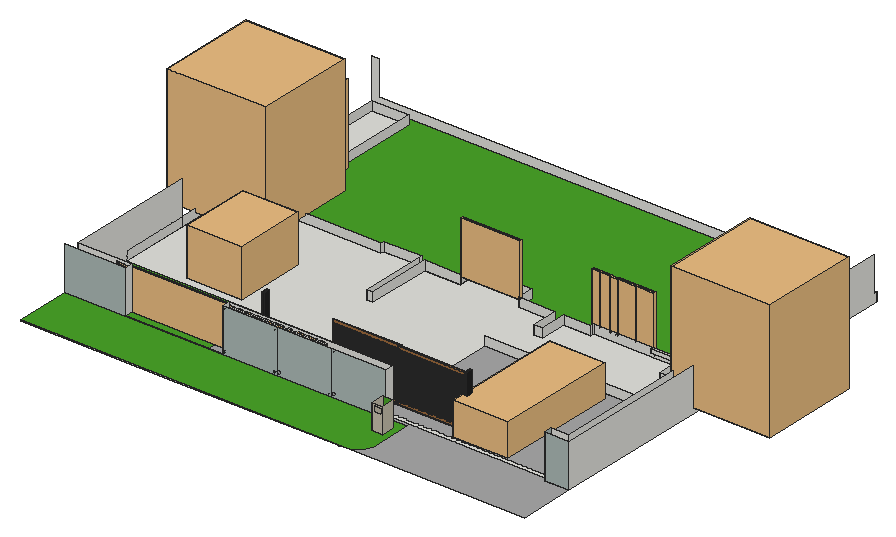
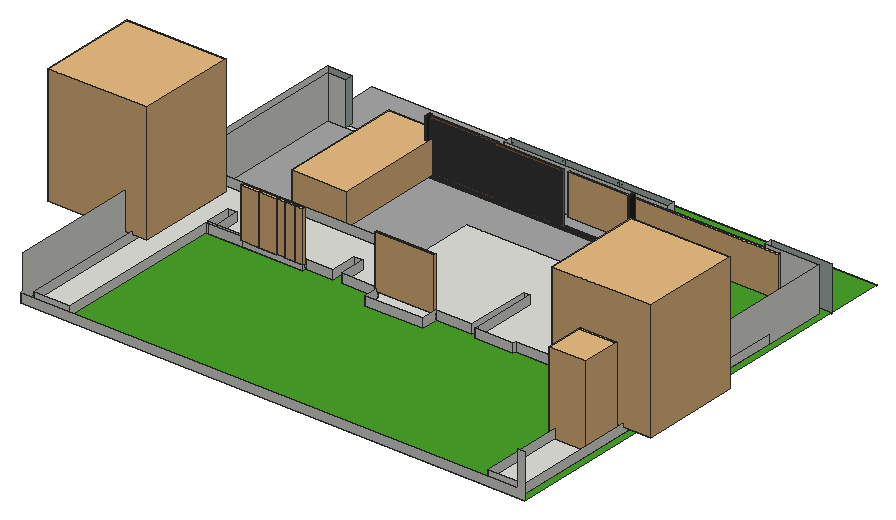
# SketchUp Ruby script. Lengths in inches.
U = 1.inch
M = Sketchup.active_model
def pt(a) = Geom::Point3d.new(a.map { |v| v * U })
def face(e, loops, mat)
  f = e.add_face(loops[0].map { |a| pt(a) })
  loops[1..].each { |l| e.add_face(l.map { |a| pt(a) }).erase! }
  f.material = f.back_material = mat if mat
  f
end
# faces: each face lists its corners as indices into pts; further lists are holes
def faces(e, pts, list, mat = nil) = list.each { |f| face(e, (f[0].is_a?(Array) ? f : [f]).map { |l| l.map { |i| pts[i] } }, mat) }
# xy, xz, yz: faces in a plane at the given z, y or x. An outline is a flat list of corners, or four numbers for a rectangle; further outlines are holes
def ring(l) = l.size == 4 ? [[l[0], l[1]], [l[2], l[1]], [l[2], l[3]], [l[0], l[3]]] : l.each_slice(2).to_a
def flat(e, list, mat, &to3) = list.each { |f| face(e, (f[0].is_a?(Array) ? f : [f]).map { |l| ring(l).map { |u, v| to3.(u, v) } }, mat) }
def xy(e, z, list, mat = nil) = flat(e, list, mat) { |x, y| [x, y, z] }
def xz(e, y, list, mat = nil) = flat(e, list, mat) { |x, z| [x, y, z] }
def yz(e, x, list, mat = nil) = flat(e, list, mat) { |y, z| [x, y, z] }
def lines(e, pts, list) = list.each { |a, b| e.add_line(pt(pts[a]), pt(pts[b])) }
# prism: a flat outline (further loops are holes) pulled along v
def prism(e, loops, v, mat = nil)
  f = face(e, loops, mat); d = Geom::Vector3d.new(v.map { |x| x * U })
  f.pushpull(f.normal.samedirection?(d) ? d.length : -d.length)
end
def box(e, o, s, mat = nil) = prism(e, [[o, [o[0] + s[0], o[1], o[2]], [o[0] + s[0], o[1] + s[1], o[2]], [o[0], o[1] + s[1], o[2]]]], [0, 0, s[2]], mat)
def at(x, y, z, deg = 0) = Geom::Transformation.translation(pt([x, y, z])) * Geom::Transformation.rotation(ORIGIN, Z_AXIS, deg.degrees)
def axes(o, x, y, z) = Geom::Transformation.new([*x, 0, *y, 0, *z, 0, *pt(o).to_a, 1])
def part(name) = M.definitions.add(name)
# library, detail: a bought-in or finely detailed component or shape, given as its bounding box
def library(name, o, s) = part(name).tap { |d| box(d.entities, o, s) }
def detail(e, o, s) = box(e.add_group.entities, o, s)
def put(e, d, t, mat = nil) = e.add_instance(d, t).tap { |i| i.material = mat if mat }
def group(e, t, mat = nil) = e.add_group.tap { |g| g.transformation = t; g.material = mat if mat }.entities
root = M.entities
M.materials.add("Material~3").color = [123, 113, 102]
M.materials.add("[0116_Lavender]").color = [73, 163, 41]
M.materials.add("[0132_LightGray]").color = [169, 169, 169]
M.materials.add("[0136_Charcoal]").color = [35, 35, 35]
M.materials.add("[Slate]").color = [172, 186, 182]
M.materials.add("[Tile Canvas]").color = [199, 192, 173]
M.materials.add("[Tile Grey]").color = [168, 168, 168]
M.materials.add("[Wood Floor Light]").color = [204, 176, 127]
M.materials.add("[Wood Floor]").color = [155, 105, 61]
c1 = library("Floor plant",[-5.56,-16.3125,0.81],[76.88,76.71,92.33])
c2 = library("Potted broadleaf plant",[-29.7,0,-10.87],[31.67,38.52,72.45])
c3 = library("Sem+nome (1)",[20.77,3.52,-2.22],[96.42,122.82,82.56])
c4 = library("Sliding Gate",[0,0,0],[194.88,4.13,70.58])
c5 = part("Group\#106")
box(c5.entities,[0,0,0],[3.9375,10.43,92.32])
c6 = library("3 door",[0,0,0],[74.8,3.9375,43.31])
c7 = part("Group\#107")
prism(c7.entities,[[[357.51,0,0.79],[357.51,0,-1.18],[357.51,10.43,-1.18],[357.51,10.43,0.79],[357.51,10.12,0.79],[357.51,10.12,0.39],[357.51,7.09,0.39],[357.51,7.09,0.79],[357.51,6.73,0.79],[357.51,6.73,0.39],[357.51,3.7,0.39],[357.51,3.7,0.79],[357.51,3.35,0.79],[357.51,3.35,0.39],[357.51,0.31,0.39],[357.51,0.31,0.79]]],[-357.51,0,0])
c8 = part("Group\#98")
box(c8.entities,[0,0,0],[1.57,1.97,82.68])
c9 = part("Group\#108")
g1 = group(c9.entities,at(0,0,0),"[Wood Floor]")
put(g1,c8,at(43.7,15.53,3.9375))
put(g1,c8,at(68.9,15.53,3.9375))
put(g1,c8,at(109.84,15.53,3.9375))
put(g1,c8,at(103.54,15.53,3.9375))
put(g1,c8,at(56.3,15.53,3.9375))
put(g1,c8,at(78.35,15.53,3.9375))
put(g1,c8,at(72.05,15.53,3.9375))
put(g1,c8,at(31.1,15.53,3.9375))
put(g1,c8,at(87.8,15.53,3.9375))
put(g1,c8,at(46.85,15.53,3.9375))
put(g1,c8,at(59.45,15.53,3.9375))
g2 = group(g1,at(12.2,15.53,3.9375))
box(g2,[0,0,0],[1.57,1.97,82.68])
put(g1,c8,at(50,15.53,3.9375))
put(g1,c8,at(106.69,15.53,3.9375))
put(g1,c8,at(34.25,15.53,3.9375))
put(g1,c8,at(81.5,15.53,3.9375))
put(g1,c8,at(53.15,15.53,3.9375))
put(g1,c8,at(27.95,15.53,3.9375))
put(g1,c8,at(65.75,15.53,3.9375))
put(g1,c8,at(18.5,15.53,3.9375))
put(g1,c8,at(40.55,15.53,3.9375))
put(g1,c8,at(75.2,15.53,3.9375))
put(g1,c8,at(21.65,15.53,3.9375))
put(g1,c8,at(62.6,15.53,3.9375))
put(g1,c8,at(84.65,15.53,3.9375))
put(g1,c8,at(100.39,15.53,3.9375))
put(g1,c8,at(112.99,15.53,3.9375))
put(g1,c8,at(24.8,15.53,3.9375))
put(g1,c8,at(37.4,15.53,3.9375))
put(g1,c8,at(97.24,15.53,3.9375))
put(g1,c8,at(2.76,15.53,3.9375))
g3 = group(g1,at(5.91,15.53,3.9375))
box(g3,[0,0,0],[1.57,1.97,82.68])
put(g1,c8,at(94.09,15.53,3.9375))
put(g1,c8,at(15.35,15.53,3.9375))
put(g1,c8,at(9.06,15.53,3.9375))
put(g1,c8,at(90.94,15.53,3.9375))
g4 = group(c9.entities,at(0,14.54,0))
xy(g4,0,[[0,0,118.11,2.95]],"[Wood Floor]")
xy(g4,3.9375,[[2.76,0,115.35,2.95]],"[Wood Floor]")
xy(g4,30.51,[[2.76,0,115.35,0.98]],"[Wood Floor]")
xy(g4,31.5,[[2.76,0,115.35,0.98]],"[Wood Floor]")
xy(g4,42.19,[[1.12,0,1.91,0.79]],"[Wood Floor]")
xy(g4,42.49,[[116.24,2.17,117.03,2.95]],"[Wood Floor]")
xy(g4,46.92,[[1.12,0,1.91,0.79]],"[Wood Floor]")
xy(g4,47.22,[[116.24,2.17,117.03,2.95]],"[Wood Floor]")
xy(g4,58.07,[[2.76,0,115.35,0.98]],"[Wood Floor Light]")
xy(g4,59.06,[[2.76,0,115.35,0.98]],"[Wood Floor]")
xy(g4,86.61,[[2.76,0,115.35,2.95]],"[Wood Floor]")
xy(g4,90.55,[[0,0,118.11,2.95]],"[Wood Floor]")
xz(g4,0,[[2.76,30.51,115.35,31.5],[2.76,58.07,115.35,59.06]],"[Wood Floor Light]")
xz(g4,0,[[[0,0,118.11,90.55],[2.76,3.9375,115.35,86.61],[1.12,42.19,1.91,46.92]]],"[Wood Floor]")
xz(g4,0.79,[[1.12,42.19,1.91,46.92]],"[Wood Floor]")
xz(g4,0.98,[[2.76,30.51,115.35,31.5],[2.76,58.07,115.35,59.06]],"[Wood Floor]")
xz(g4,2.17,[[116.24,42.49,117.03,47.22]],"[Wood Floor]")
xz(g4,2.95,[[[0,0,118.11,90.55],[2.76,3.9375,115.35,86.61],[116.24,42.49,117.03,47.22]]],"[Wood Floor]")
yz(g4,0,[[0,0,2.95,90.55]],"[Wood Floor]")
yz(g4,1.12,[[0,42.19,0.79,46.92]],"[Wood Floor]")
yz(g4,1.91,[[0,42.19,0.79,46.92]],"[Wood Floor]")
yz(g4,2.76,[[0,3.9375,2.95,3.9375,2.95,86.61,0,86.61,0,59.06,0.98,59.06,0.98,58.07,0,58.07,0,31.5,0.98,31.5,0.98,30.51,0,30.51],[0,30.51,0.98,31.5],[0,58.07,0.98,59.06]],"[Wood Floor]")
yz(g4,115.35,[[0,3.9375,0,30.51,0.98,30.51,0.98,31.5,0,31.5,0,58.07,0.98,58.07,0.98,59.06,0,59.06,0,86.61,2.95,86.61,2.95,3.9375],[0,30.51,0.98,31.5],[0,58.07,0.98,59.06]],"[Wood Floor]")
yz(g4,116.24,[[2.17,42.49,2.95,47.22]],"[Wood Floor]")
yz(g4,117.03,[[2.17,42.49,2.95,47.22]],"[Wood Floor]")
yz(g4,118.11,[[0,0,2.95,90.55]],"[Wood Floor]")
p = [[5.91,2.95,86.61],[5.91,2.95,3.9375]]
lines(g4,p,[[0,1]])
c10 = part("Group\#103")
put(c10.entities,c8,at(43.7,15.53,3.9375))
put(c10.entities,c8,at(68.9,15.53,3.9375))
put(c10.entities,c8,at(109.84,15.53,3.9375))
put(c10.entities,c8,at(103.54,15.53,3.9375))
put(c10.entities,c8,at(56.3,15.53,3.9375))
put(c10.entities,c8,at(78.35,15.53,3.9375))
put(c10.entities,c8,at(72.05,15.53,3.9375))
put(c10.entities,c8,at(31.1,15.53,3.9375))
put(c10.entities,c8,at(87.8,15.53,3.9375))
put(c10.entities,c8,at(46.85,15.53,3.9375))
put(c10.entities,c8,at(59.45,15.53,3.9375))
put(c10.entities,c8,at(12.2,15.53,3.9375))
put(c10.entities,c8,at(50,15.53,3.9375))
put(c10.entities,c8,at(106.69,15.53,3.9375))
put(c10.entities,c8,at(34.25,15.53,3.9375))
put(c10.entities,c8,at(81.5,15.53,3.9375))
put(c10.entities,c8,at(53.15,15.53,3.9375))
put(c10.entities,c8,at(27.95,15.53,3.9375))
put(c10.entities,c8,at(65.75,15.53,3.9375))
put(c10.entities,c8,at(18.5,15.53,3.9375))
put(c10.entities,c8,at(40.55,15.53,3.9375))
put(c10.entities,c8,at(75.2,15.53,3.9375))
put(c10.entities,c8,at(21.65,15.53,3.9375))
put(c10.entities,c8,at(62.6,15.53,3.9375))
put(c10.entities,c8,at(84.65,15.53,3.9375))
put(c10.entities,c8,at(100.39,15.53,3.9375))
put(c10.entities,c8,at(112.99,15.53,3.9375))
put(c10.entities,c8,at(24.8,15.53,3.9375))
put(c10.entities,c8,at(37.4,15.53,3.9375))
put(c10.entities,c8,at(97.24,15.53,3.9375))
put(c10.entities,c8,at(2.76,15.53,3.9375))
put(c10.entities,c8,at(5.91,15.53,3.9375))
put(c10.entities,c8,at(94.09,15.53,3.9375))
put(c10.entities,c8,at(15.35,15.53,3.9375))
put(c10.entities,c8,at(9.06,15.53,3.9375))
put(c10.entities,c8,at(90.94,15.53,3.9375))
c11 = part("Group\#104")
put(c11.entities,c10,at(0,0,0),"[Wood Floor]")
g5 = group(c11.entities,at(0,14.54,0))
xy(g5,0,[[0,0,118.11,2.95]],"[Wood Floor]")
xy(g5,3.9375,[[2.76,0,115.35,2.95]],"[Wood Floor]")
xy(g5,30.51,[[2.76,0,115.35,0.98]],"[Wood Floor]")
xy(g5,31.5,[[2.76,0,115.35,0.98]],"[Wood Floor]")
xy(g5,42.07,[[116.14,2.17,116.92,2.95]],"[Wood Floor]")
xy(g5,42.125,[[1.06,0,1.84,0.79]],"[Wood Floor]")
xy(g5,46.8,[[116.14,2.17,116.92,2.95]],"[Wood Floor]")
xy(g5,46.85,[[1.06,0,1.84,0.79]],"[Wood Floor]")
xy(g5,58.07,[[2.76,0,115.35,0.98]],"[Wood Floor Light]")
xy(g5,59.06,[[2.76,0,115.35,0.98]],"[Wood Floor]")
xy(g5,86.61,[[2.76,0,115.35,2.95]],"[Wood Floor]")
xy(g5,90.55,[[0,0,118.11,2.95]],"[Wood Floor]")
xz(g5,0,[[2.76,30.51,115.35,31.5],[2.76,58.07,115.35,59.06]],"[Wood Floor Light]")
xz(g5,0,[[[0,0,118.11,90.55],[2.76,3.9375,115.35,86.61],[1.06,42.125,1.84,46.85]]],"[Wood Floor]")
xz(g5,0.79,[[1.06,42.125,1.84,46.85]],"[Wood Floor]")
xz(g5,0.98,[[2.76,30.51,115.35,31.5],[2.76,58.07,115.35,59.06]],"[Wood Floor]")
xz(g5,2.17,[[116.14,42.07,116.92,46.8]],"[Wood Floor]")
xz(g5,2.95,[[[0,0,118.11,90.55],[2.76,3.9375,115.35,86.61],[116.14,42.07,116.92,46.8]]],"[Wood Floor]")
yz(g5,0,[[0,0,2.95,90.55]],"[Wood Floor]")
yz(g5,1.06,[[0,42.125,0.79,46.85]],"[Wood Floor]")
yz(g5,1.84,[[0,42.125,0.79,46.85]],"[Wood Floor]")
yz(g5,2.76,[[0,3.9375,2.95,3.9375,2.95,86.61,0,86.61,0,59.06,0.98,59.06,0.98,58.07,0,58.07,0,31.5,0.98,31.5,0.98,30.51,0,30.51],[0,30.51,0.98,31.5],[0,58.07,0.98,59.06]],"[Wood Floor]")
yz(g5,115.35,[[0,3.9375,0,30.51,0.98,30.51,0.98,31.5,0,31.5,0,58.07,0.98,58.07,0.98,59.06,0,59.06,0,86.61,2.95,86.61,2.95,3.9375],[0,30.51,0.98,31.5],[0,58.07,0.98,59.06]],"[Wood Floor]")
yz(g5,116.14,[[2.17,42.07,2.95,46.8]],"[Wood Floor]")
yz(g5,116.92,[[2.17,42.07,2.95,46.8]],"[Wood Floor]")
yz(g5,118.11,[[0,0,2.95,90.55]],"[Wood Floor]")
p = [[5.91,2.95,86.61],[5.91,2.95,3.9375]]
lines(g5,p,[[0,1]])
c12 = library("3DGeom~4_Defintion",[362.52,-15.59,12.6],[288.85,70.11,1000])
c13 = library("BMW 8 Series M850i 2019",[-14.25,0.77,-0.16],[87.38,190.63,50.87])
xy(root,-10.51,[[3476.5,498.28,3753.3125,505.1],[[2928.38,611.53,2928.38,1146.63,2992.01,1146.63,2992.01,732.28,3002.95,732.28,3002.95,845.35,3184.99,845.35,3184.99,851.0625,3250.36,851.0625,3250.36,732.28,3261.3,732.28,3261.3,845.35,3323.99,845.35,3323.99,874.25,3424.27,874.25,3424.27,845.35,3488.55,845.35,3488.55,798.41,3503.88,798.41,3503.88,845.35,3551.34,845.35,3551.34,851.0625,3720.76,851.0625,3720.76,1146.63,3784.01,1146.63,3784.01,732.28,3456.29,732.28,3456.29,611.53],[3705.43,801.78,3720.76,845.35]]])
xy(root,-10.51,[[[2916.76,393.78,3487,393.78,3490.03,394.71,3492.96,395.9,3495.78,397.35,3498.46,399.04,3500.97,400.97,3503.31,403.1,3505.45,405.44,3507.37,407.96,3509.06,410.63,3510.51,413.45,3511.7,416.38,3512.63,419.41,3512.63,491.47,3476.5,491.47,3476.5,505.1,3191.65,505.1,3191.65,491.47,3022.65,491.47,3022.65,505.1,2928.38,505.1,2928.38,1146.63,2992.01,1146.63,2992.01,732.28,3002.95,732.28,3002.95,845.35,3184.99,845.35,3184.99,851.0625,3250.36,851.0625,3250.36,732.28,3261.3,732.28,3261.3,845.35,3323.99,845.35,3323.99,874.25,3424.27,874.25,3424.27,845.35,3488.55,845.35,3488.55,798.41,3503.88,798.41,3503.88,845.35,3551.34,845.35,3551.34,851.0625,3720.76,851.0625,3720.76,1146.63,3784.01,1146.63,3784.01,505.1,3753.3125,505.1,3753.3125,491.47,3796.01,491.47,3796.01,1160.85,2916.76,1160.85],[3482.52,453.42,3500.96,475.99]],[3022.65,491.47,3166.09,491.47,3171.29,611.53,2928.38,611.53,2928.38,505.1,3022.65,505.1]],"[0116_Lavender]")
xy(root,-10.51,[[3487,393.78,3796.01,393.78,3796.01,491.47,3753.3125,491.47,3753.3125,498.28,3476.5,498.28,3476.5,491.47,3512.63,491.47,3512.63,419.41,3511.7,416.38,3510.51,413.45,3509.06,410.63,3507.37,407.96,3505.45,405.44,3503.31,403.1,3500.97,400.97,3498.46,399.04,3495.78,397.35,3492.96,395.9,3490.03,394.71],[3166.09,491.47,3191.65,491.47,3191.65,505.1,3784.01,505.1,3784.01,732.28,3456.29,732.28,3456.29,611.53,3171.29,611.53]],"[Tile Grey]")
xz(root,393.78,[[2916.76,-12.6875,3191.65,-12.6875,3476.5,-10.51,2916.76,-10.51]])
xz(root,453.42,[[[3482.52,-10.51,3500.96,32.74],[3484.87,19.53,3499,29.34]]],"[Tile Canvas]")
xz(root,475.99,[[3482.52,-10.51,3500.96,32.74]],"[0116_Lavender]")
xz(root,491.47,[[3022.65,-12.6875,3191.65,-10.51]])
xz(root,491.47,[[3282.87,-7.89,3283.35,-7.82,3283.8,-7.63,3284.19,-7.34,3284.49,-6.95,3284.68,-6.5,3284.74,-6.01,3284.68,-5.52,3284.49,-5.07,3284.19,-4.68,3283.8,-4.39,3283.35,-4.2,3282.87,-4.14,3282.38,-4.2,3281.93,-4.39,3281.54,-4.68,3281.24,-5.07,3281.06,-5.52,3280.99,-6.01,3281.06,-6.5,3281.24,-6.95,3281.54,-7.34,3281.93,-7.63,3282.38,-7.82],[3377.82,-7.89,3378.3,-7.82,3378.76,-7.63,3379.14,-7.34,3379.44,-6.95,3379.63,-6.5,3379.69,-6.01,3379.63,-5.52,3379.44,-5.07,3379.14,-4.68,3378.76,-4.39,3378.3,-4.2,3377.82,-4.14,3377.33,-4.2,3376.88,-4.39,3376.49,-4.68,3376.19,-5.07,3376.01,-5.52,3375.94,-6.01,3376.01,-6.5,3376.19,-6.95,3376.49,-7.34,3376.88,-7.63,3377.33,-7.82],[3472.77,-7.89,3473.25,-7.82,3473.71,-7.63,3474.09,-7.34,3474.39,-6.95,3474.58,-6.5,3474.64,-6.01,3474.58,-5.52,3474.39,-5.07,3474.09,-4.68,3473.71,-4.39,3473.25,-4.2,3472.77,-4.14,3472.28,-4.2,3471.83,-4.39,3471.44,-4.68,3471.15,-5.07,3470.96,-5.52,3470.89,-6.01,3470.96,-6.5,3471.15,-6.95,3471.44,-7.34,3471.83,-7.63,3472.28,-7.82],[3195.13,-6.41,3195.625,-6.4,3196.09,-6.26,3196.51,-6.01,3196.85,-5.66,3197.08,-5.23,3197.2,-4.75,3197.1875,-4.26,3197.05,-3.79,3196.79,-3.375,3196.4375,-3.04,3196.01,-2.8,3195.53,-2.6875,3195.04,-2.7,3194.57,-2.84,3194.16,-3.09,3193.82,-3.45,3193.58,-3.875,3193.47,-4.35,3193.48,-4.84,3193.62,-5.31,3193.875,-5.73,3194.23,-6.07,3194.66,-6.3],[3290.09,-6.41,3290.57,-6.4,3291.04,-6.26,3291.46,-6.01,3291.8,-5.66,3292.03,-5.23,3292.15,-4.75,3292.14,-4.26,3292,-3.79,3291.74,-3.375,3291.39,-3.04,3290.96,-2.8,3290.48,-2.6875,3290,-2.7,3289.53,-2.84,3289.11,-3.09,3288.77,-3.45,3288.54,-3.875,3288.42,-4.35,3288.43,-4.84,3288.57,-5.31,3288.83,-5.73,3289.18,-6.07,3289.61,-6.3],
  [3385.04,-6.41,3385.53,-6.4,3385.99,-6.26,3386.41,-6.01,3386.75,-5.66,3386.98,-5.23,3387.1,-4.75,3387.09,-4.26,3386.95,-3.79,3386.7,-3.375,3386.34,-3.04,3385.91,-2.8,3385.44,-2.6875,3384.95,-2.7,3384.48,-2.84,3384.06,-3.09,3383.72,-3.45,3383.49,-3.875,3383.37,-4.35,3383.38,-4.84,3383.52,-5.31,3383.78,-5.73,3384.13,-6.07,3384.56,-6.3]],"[0132_LightGray]")
xz(root,491.47,[[2916.76,-12.6875,3022.65,65.1875],[[3191.65,-12.6875,3476.5,-10.51,3476.5,65.1875,3191.65,65.1875],[3282.87,-7.89,3282.38,-7.82,3281.93,-7.63,3281.54,-7.34,3281.24,-6.95,3281.06,-6.5,3280.99,-6.01,3281.06,-5.52,3281.24,-5.07,3281.54,-4.68,3281.93,-4.39,3282.38,-4.2,3282.87,-4.14,3283.35,-4.2,3283.8,-4.39,3284.19,-4.68,3284.49,-5.07,3284.68,-5.52,3284.74,-6.01,3284.68,-6.5,3284.49,-6.95,3284.19,-7.34,3283.8,-7.63,3283.35,-7.82],[3377.82,-7.89,3377.33,-7.82,3376.88,-7.63,3376.49,-7.34,3376.19,-6.95,3376.01,-6.5,3375.94,-6.01,3376.01,-5.52,3376.19,-5.07,3376.49,-4.68,3376.88,-4.39,3377.33,-4.2,3377.82,-4.14,3378.3,-4.2,3378.76,-4.39,3379.14,-4.68,3379.44,-5.07,3379.63,-5.52,3379.69,-6.01,3379.63,-6.5,3379.44,-6.95,3379.14,-7.34,3378.76,-7.63,3378.3,-7.82],[3282.87,57.74,3282.38,57.8,3281.93,57.99,3281.54,58.29,3281.24,58.68,3281.06,59.13,3280.99,59.61,3281.06,60.1,3281.24,60.55,3281.54,60.94,3281.93,61.24,3282.38,61.43,3282.87,61.49,3283.35,61.43,3283.8,61.24,3284.19,60.94,3284.49,60.55,3284.68,60.1,3284.74,59.61,3284.68,59.13,3284.49,58.68,3284.19,58.29,3283.8,57.99,3283.35,57.8],[3377.82,57.74,3377.33,57.8,3376.88,57.99,3376.49,58.29,3376.19,58.68,3376.01,59.13,3375.94,59.61,3376.01,60.1,3376.19,60.55,3376.49,60.94,3376.88,61.24,3377.33,61.43,3377.82,61.49,3378.3,61.43,3378.76,61.24,3379.14,60.94,3379.44,60.55,3379.63,60.1,3379.69,59.61,3379.63,59.13,3379.44,58.68,3379.14,58.29,3378.76,57.99,3378.3,57.8],[3472.77,-7.89,3472.28,-7.82,3471.83,-7.63,3471.44,-7.34,3471.15,-6.95,3470.96,-6.5,3470.89,-6.01,3470.96,-5.52,3471.15,-5.07,3471.44,-4.68,3471.83,-4.39,3472.28,-4.2,3472.77,-4.14,3473.25,-4.2,3473.71,-4.39,3474.09,-4.68,3474.39,-5.07,3474.58,-5.52,3474.64,-6.01,3474.58,-6.5,3474.39,-6.95,3474.09,-7.34,3473.71,-7.63,3473.25,-7.82],[3472.77,57.74,3472.28,57.8,3471.83,57.99,3471.44,58.29,3471.15,58.68,3470.96,59.13,3470.89,59.61,3470.96,60.1,3471.15,60.55,3471.44,60.94,3471.83,61.24,3472.28,61.43,3472.77,61.49,3473.25,61.43,3473.71,61.24,3474.09,60.94,3474.39,60.55,3474.58,60.1,3474.64,59.61,3474.58,59.13,3474.39,58.68,3474.09,58.29,3473.71,57.99,3473.25,57.8],[3290.09,59.21,3289.61,59.33,3289.18,59.56,3288.83,59.9,3288.57,60.32,3288.43,60.78,3288.42,61.27,3288.54,61.75,3288.77,62.18,3289.11,62.53,3289.53,62.79,3290,62.93,3290.48,62.9375,3290.96,62.82,3291.39,62.59,3291.74,62.25,3292,61.83,3292.14,61.36,3292.15,60.875,3292.03,60.4,3291.8,59.97,3291.46,59.61,3291.04,59.36,3290.57,59.22],[3385.04,59.21,3384.56,59.33,3384.13,59.56,3383.78,59.9,3383.52,60.32,3383.38,60.78,3383.37,61.27,3383.49,61.75,3383.72,62.18,3384.06,62.53,3384.48,62.79,3384.95,62.93,3385.44,62.9375,3385.91,62.82,3386.34,62.59,3386.7,62.25,3386.95,61.83,3387.09,61.36,3387.1,60.875,3386.98,60.4,3386.75,59.97,3386.41,59.61,3385.99,59.36,3385.53,59.22],[3195.13,-6.41,3194.66,-6.3,3194.23,-6.07,3193.875,-5.73,3193.62,-5.31,3193.48,-4.84,3193.47,-4.35,3193.58,-3.875,3193.82,-3.45,3194.16,-3.09,3194.57,-2.84,3195.04,-2.7,3195.53,-2.6875,3196.01,-2.8,3196.4375,-3.04,3196.79,-3.375,3197.05,-3.79,3197.1875,-4.26,3197.2,-4.75,3197.08,-5.23,3196.85,-5.66,3196.51,-6.01,3196.09,-6.26,3195.625,-6.4],[3290.09,-6.41,3289.61,-6.3,3289.18,-6.07,3288.83,-5.73,3288.57,-5.31,3288.43,-4.84,3288.42,-4.35,3288.54,-3.875,3288.77,-3.45,3289.11,-3.09,3289.53,-2.84,3290,-2.7,3290.48,-2.6875,3290.96,-2.8,3291.39,-3.04,3291.74,-3.375,3292,-3.79,3292.14,-4.26,3292.15,-4.75,3292.03,-5.23,3291.8,-5.66,3291.46,-6.01,3291.04,-6.26,3290.57,-6.4],[3385.04,-6.41,3384.56,-6.3,3384.13,-6.07,3383.78,-5.73,3383.52,-5.31,3383.38,-4.84,3383.37,-4.35,3383.49,-3.875,3383.72,-3.45,3384.06,-3.09,3384.48,-2.84,3384.95,-2.7,3385.44,-2.6875,3385.91,-2.8,3386.34,-3.04,3386.7,-3.375,3386.95,-3.79,3387.09,-4.26,3387.1,-4.75,3386.98,-5.23,3386.75,-5.66,3386.41,-6.01,3385.99,-6.26,3385.53,-6.4],[3195.13,59.21,3194.66,59.33,3194.23,59.56,3193.875,59.9,3193.62,60.32,3193.48,60.78,3193.47,61.27,3193.58,61.75,3193.82,62.18,3194.16,62.53,3194.57,62.79,3195.04,62.93,3195.53,62.9375,3196.01,62.82,3196.4375,62.59,3196.79,62.25,3197.05,61.83,3197.1875,61.36,3197.2,60.875,3197.08,60.4,3196.85,59.97,3196.51,59.61,3196.09,59.36,3195.625,59.22]],[3753.3125,-10.51,3796.01,65.1875]],"[Slate]")
xz(root,505.1,[[2928.38,-10.51,3022.65,65.1875],[3191.65,-10.51,3476.5,65.1875],[3753.3125,-10.51,3784.01,65.1875]])
xz(root,732.28,[[2992.01,-10.51,3002.95,5.1875],[3250.36,-10.51,3261.3,5.1875],[3456.29,-10.51,3784.01,5.1875]])
xz(root,798.41,[[3488.55,-10.51,3503.88,5.1875]])
xz(root,801.78,[[3705.43,-10.51,3720.76,5.1875]])
xz(root,845.35,[[3002.95,-10.51,3184.99,5.1875],[3261.3,-10.51,3323.99,5.1875],[3424.27,-10.51,3488.55,5.1875],[3503.88,-10.51,3551.34,5.1875],[3705.43,-10.51,3720.76,5.1875],
  [3655.96,-0.125,3705.43,5.1875]])
xz(root,851.0625,[[3184.99,-10.51,3250.36,5.1875],[3551.34,-10.51,3655.96,5.1875],[3655.96,-10.51,3715.04,5.1875],[3715.04,-10.51,3720.76,5.1875]])
xz(root,874.25,[[3323.99,-10.51,3424.27,5.1875]])
xz(root,1146.63,[[2928.38,-10.51,2992.01,5.1875],[3720.76,-10.51,3784.01,5.1875]])
xz(root,1160.85,[[2916.76,-10.51,2916.76,65.1875,2928.38,65.1875,2928.38,5.1875,3796.01,5.1875,3796.01,-10.51]])
yz(root,2928.38,[[505.1,-10.51,611.53,-10.51,611.53,5.1875,732.28,5.1875,732.28,65.1875,505.1,65.1875],[611.53,-10.51,732.28,5.1875],[732.28,-10.51,1146.63,5.1875]])
yz(root,2992.01,[[732.28,-10.51,1146.63,5.1875]])
yz(root,3002.95,[[732.28,-10.51,845.35,5.1875]])
yz(root,3022.65,[[491.47,-10.51,505.1,65.1875]])
yz(root,3184.99,[[845.35,-10.51,851.0625,5.1875]])
yz(root,3191.65,[[491.47,-10.51,505.1,65.1875]])
yz(root,3250.36,[[732.28,-10.51,846.1,5.1875],[846.1,-10.51,851.0625,5.1875]])
yz(root,3261.3,[[732.28,-10.51,845.35,5.1875]])
yz(root,3323.99,[[845.35,-10.51,846.1,5.1875],[846.1,-10.51,874.25,5.1875]])
yz(root,3424.27,[[845.35,-10.51,846.1,5.1875],[846.1,-10.51,874.25,5.1875]])
yz(root,3476.5,[[491.47,-10.51,505.1,65.1875]])
yz(root,3482.52,[[453.42,-10.51,475.99,32.74]],"[Tile Canvas]")
yz(root,3488.55,[[798.41,-10.51,845.35,5.1875]])
yz(root,3500.96,[[453.42,-10.51,475.99,32.74]],"[Tile Canvas]")
yz(root,3503.88,[[798.41,-10.51,845.35,5.1875]])
yz(root,3551.34,[[845.35,-10.51,846.1,5.1875],[846.1,-10.51,851.0625,5.1875]])
yz(root,3655.96,[[845.35,-0.125,851.0625,5.1875]])
yz(root,3705.43,[[801.78,-10.51,845.35,5.1875]])
yz(root,3720.76,[[801.78,-10.51,845.35,5.1875],[851.0625,-10.51,1146.63,5.1875]])
yz(root,3753.3125,[[491.47,-10.51,505.1,65.1875]],"[Slate]")
yz(root,3784.01,[[505.1,-10.51,732.28,65.1875],[732.28,-10.51,1146.63,5.1875]])
yz(root,3796.01,[[491.47,-10.51,1160.85,-10.51,1160.85,5.1875,1155.13,5.1875,1155.13,65.1875,491.47,65.1875]])
p = [[3466.9375,532.58,-10.51],[3465.8,532.58,-10.51],[3286.6,491.47,65.1875],[3286.6,491.47,-10.51],[3381.55,491.47,65.1875],[3381.55,491.47,-10.51]]
lines(root,p,[[0,1],[2,3],[4,5]])
put(root,c1,axes([2891.18,797.14,-1],[2.24,0,0],[0,2.24,0],[0,0,2.24]))
put(root,c2,axes([2997.64,858.27,6.22],[2,0,0],[0,2,0],[0,0,2]))
put(root,c2,axes([2997.64,924.09,6.22],[2,0,0],[0,2,0],[0,0,2]))
put(root,c3,at(3008.77,611.53,-0.125))
put(root,c4,axes([2995.21,505.1,-10.51],[1.88,0,0],[0,1,0],[0,0,1]))
put(root,c5,at(3229.18,530.57,-10.11),"[0136_Charcoal]")
put(root,c6,axes([3323.99,846.14,1.53],[1.37387,0,0],[0,0.86071,0],[0,0,2.11056]))
put(root,c7,at(3229.18,530.57,-10.51),"[0136_Charcoal]")
put(root,c9,at(3349.21,519.73,-10.11))
put(root,c11,at(3464.57,516.42,-9.72))
put(root,c12,axes([3507.63,854.26,0.98],[0.11056,0,0],[0,-0.05859,0],[0,0,0.08734]),"Material~3")
put(root,c12,axes([3521.68,854.26,0.98],[0.11056,0,0],[0,-0.05859,0],[0,0,0.08734]),"Material~3")
put(root,c5,at(3582.76,530.57,-10.11),"[0136_Charcoal]")
put(root,c12,axes([3552.26,854.26,0.98],[0.11056,0,0],[0,-0.05859,0],[0,0,0.08734]),"Material~3")
put(root,c13,axes([3659.99,720.81,-10.33],[-1.11,0,0],[0,-1.11,0],[0,0,1.11]))
put(root,c12,axes([3583.94,854.26,0.98],[0.11056,0,0],[0,-0.05859,0],[0,0,0.08734]),"Material~3")
put(root,c1,axes([3771.12,797.14,-1],[2.24,0,0],[0,2.24,0],[0,0,2.24]))
